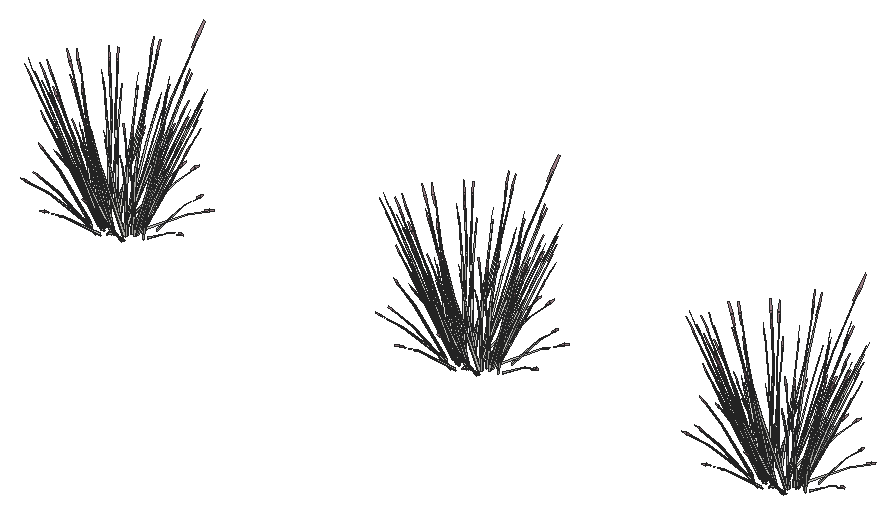
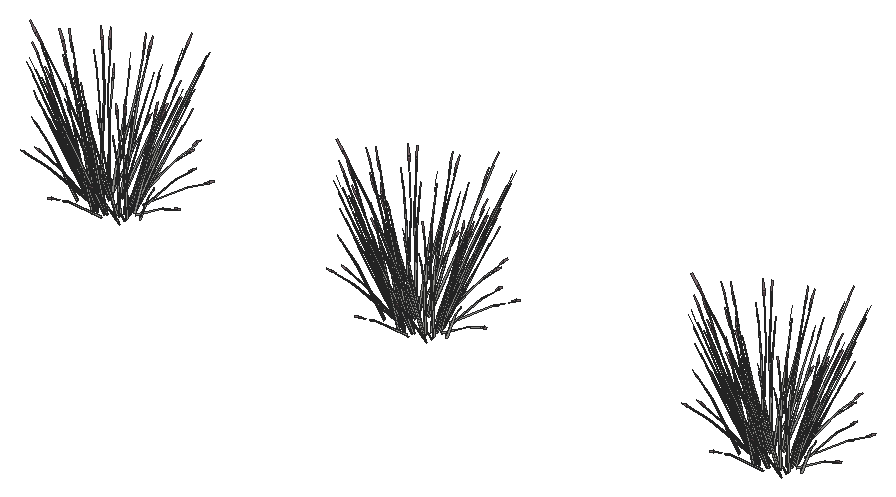
# SketchUp Ruby script. Lengths in millimetres.
U = 1.mm
M = Sketchup.active_model
def pt(a) = Geom::Point3d.new(a.map { |v| v * U })
def face(e, loops, mat)
  f = e.add_face(loops[0].map { |a| pt(a) })
  loops[1..].each { |l| e.add_face(l.map { |a| pt(a) }).erase! }
  f.material = f.back_material = mat if mat
  f
end
# faces: each face lists its corners as indices into pts; further lists are holes
def faces(e, pts, list, mat = nil) = list.each { |f| face(e, (f[0].is_a?(Array) ? f : [f]).map { |l| l.map { |i| pts[i] } }, mat) }
# xy, xz, yz: faces in a plane at the given z, y or x. An outline is a flat list of corners, or four numbers for a rectangle; further outlines are holes
def ring(l) = l.size == 4 ? [[l[0], l[1]], [l[2], l[1]], [l[2], l[3]], [l[0], l[3]]] : l.each_slice(2).to_a
def flat(e, list, mat, &to3) = list.each { |f| face(e, (f[0].is_a?(Array) ? f : [f]).map { |l| ring(l).map { |u, v| to3.(u, v) } }, mat) }
def xy(e, z, list, mat = nil) = flat(e, list, mat) { |x, y| [x, y, z] }
def xz(e, y, list, mat = nil) = flat(e, list, mat) { |x, z| [x, y, z] }
def yz(e, x, list, mat = nil) = flat(e, list, mat) { |y, z| [x, y, z] }
def lines(e, pts, list) = list.each { |a, b| e.add_line(pt(pts[a]), pt(pts[b])) }
# prism: a flat outline (further loops are holes) pulled along v
def prism(e, loops, v, mat = nil)
  f = face(e, loops, mat); d = Geom::Vector3d.new(v.map { |x| x * U })
  f.pushpull(f.normal.samedirection?(d) ? d.length : -d.length)
end
def box(e, o, s, mat = nil) = prism(e, [[o, [o[0] + s[0], o[1], o[2]], [o[0] + s[0], o[1] + s[1], o[2]], [o[0], o[1] + s[1], o[2]]]], [0, 0, s[2]], mat)
def at(x, y, z, deg = 0) = Geom::Transformation.translation(pt([x, y, z])) * Geom::Transformation.rotation(ORIGIN, Z_AXIS, deg.degrees)
def axes(o, x, y, z) = Geom::Transformation.new([*x, 0, *y, 0, *z, 0, *pt(o).to_a, 1])
def part(name) = M.definitions.add(name)
# library, detail: a bought-in or finely detailed component or shape, given as its bounding box
def library(name, o, s) = part(name).tap { |d| box(d.entities, o, s) }
def detail(e, o, s) = box(e.add_group.entities, o, s)
def put(e, d, t, mat = nil) = e.add_instance(d, t).tap { |i| i.material = mat if mat }
def group(e, t, mat = nil) = e.add_group.tap { |g| g.transformation = t; g.material = mat if mat }.entities
root = M.entities
M.materials.add("LightPink_Translucent").color = [144, 107, 117]
M.materials["LightPink_Translucent"].alpha = 0.8
c1 = part("blade")
p = [[54.7,5.3,558.8],[0,4.4,0],[2.3,11.5,0],[55.5,7.8,558.8],[58.2,7.8,558.8],[9.8,11.5,0],
  [62.9,5.7,838.2],[63,6,838.2],[63.4,6,838.2]]
faces(c1.entities,p,[[0,1,2,3],[4,5,2,3],[6,0,3,7],[7,3,4,8]])
c2 = part("seeds")
p = [[7.6,-2.7,35.1],[-0.2,-0.6,40.4],[-0.2,-0.8,0.9],[3.5,-1.8,-1.7],[7.5,-0.8,76.3],[3.7,0.2,78.9]]
faces(c2.entities,p,[[0,1,2,3],[1,0,4,5]],"LightPink_Translucent")
c3 = part("blade with seeds")
put(c3.entities,c1,at(0,0,0))
put(c3.entities,c2,axes([60.9,6.5,787.2],[1.5799,-0.05474,1.17369],[-0.12525,1.92788,0.29478],[-0.07173,-0.02425,1.56792]))
put(root,c3,axes([12521.7,4405.6,127.9],[0.06562,-1.05324,-0.1216],[1.2424,0.02879,-0.67495],[0.4785,0.07316,1.02557]))
put(root,c3,axes([12285.5,4303,127.9],[0.6166,0.93779,-0.1216],[-1.09436,0.46085,-0.67495],[-0.46117,0.12373,1.02557]))
put(root,c3,axes([12518.5,4251,127.9],[-1.34686,-0.05131,-0.1216],[0.03681,-0.97156,-0.67495],[0.09356,-0.37418,1.02557]))
put(root,c3,axes([12556.8,4356.2,127.9],[-0.6166,-0.93779,-0.1216],[1.09436,-0.46085,-0.67495],[0.46117,-0.12373,1.02557]))
put(root,c3,axes([12387.1,4435.7,127.9],[1.19922,-0.48218,-0.1216],[0.58932,0.85579,-0.67495],[0.15822,0.36063,1.02557]))
put(root,c3,axes([12320.7,4253.5,127.9],[-0.06562,1.05324,-0.1216],[-1.2424,-0.02879,-0.67495],[-0.4785,-0.07316,1.02557]))
put(root,c3,axes([12459.5,4434.8,127.9],[0.73026,-0.88648,-0.1216],[1.05755,0.51071,-0.67495],[0.36761,0.25045,1.02557]))
put(root,c3,axes([12286.7,4359.6,127.9],[1.1336,0.57106,-0.1216],[-0.65308,0.827,-0.67495],[-0.32027,0.28747,1.02557]))
put(root,c3,axes([12455.2,4223.5,127.9],[-1.19922,0.48218,-0.1216],[-0.58932,-0.85579,-0.67495],[-0.15822,-0.36063,1.02557]))
put(root,c3,axes([12555.7,4299.5,127.9],[-1.1336,-0.57106,-0.1216],[0.65308,-0.827,-0.67495],[0.32027,-0.28747,1.02557]))
put(root,c3,axes([10242,4389.4,127.9],[0.06562,-1.05324,-0.1216],[1.2424,0.02879,-0.67495],[0.4785,0.07316,1.02557]))
put(root,c3,axes([10005.8,4286.7,127.9],[0.6166,0.93779,-0.1216],[-1.09436,0.46085,-0.67495],[-0.46117,0.12373,1.02557]))
put(root,c3,axes([10238.8,4234.8,127.9],[-1.34686,-0.05131,-0.1216],[0.03681,-0.97156,-0.67495],[0.09356,-0.37418,1.02557]))
put(root,c3,axes([10277.2,4339.9,127.9],[-0.6166,-0.93779,-0.1216],[1.09436,-0.46085,-0.67495],[0.46117,-0.12373,1.02557]))
put(root,c3,axes([10107.5,4419.4,127.9],[1.19922,-0.48218,-0.1216],[0.58932,0.85579,-0.67495],[0.15822,0.36063,1.02557]))
put(root,c3,axes([10041,4237.3,127.9],[-0.06562,1.05324,-0.1216],[-1.2424,-0.02879,-0.67495],[-0.4785,-0.07316,1.02557]))
put(root,c3,axes([10179.9,4418.5,127.9],[0.73026,-0.88648,-0.1216],[1.05755,0.51071,-0.67495],[0.36761,0.25045,1.02557]))
put(root,c3,axes([10007,4343.4,127.9],[1.1336,0.57106,-0.1216],[-0.65308,0.827,-0.67495],[-0.32027,0.28747,1.02557]))
put(root,c3,axes([10175.5,4207.2,127.9],[-1.19922,0.48218,-0.1216],[-0.58932,-0.85579,-0.67495],[-0.15822,-0.36063,1.02557]))
put(root,c3,axes([10276,4283.3,127.9],[-1.1336,-0.57106,-0.1216],[0.65308,-0.827,-0.67495],[0.32027,-0.28747,1.02557]))
put(root,c3,axes([7622,4346,127.9],[0.06562,-1.05324,-0.1216],[1.2424,0.02879,-0.67495],[0.4785,0.07316,1.02557]))
put(root,c3,axes([7385.8,4243.3,127.9],[0.6166,0.93779,-0.1216],[-1.09436,0.46085,-0.67495],[-0.46117,0.12373,1.02557]))
put(root,c3,axes([7618.8,4191.3,127.9],[-1.34686,-0.05131,-0.1216],[0.03681,-0.97156,-0.67495],[0.09356,-0.37418,1.02557]))
put(root,c3,axes([7657.2,4296.5,127.9],[-0.6166,-0.93779,-0.1216],[1.09436,-0.46085,-0.67495],[0.46117,-0.12373,1.02557]))
put(root,c3,axes([7487.5,4376,127.9],[1.19922,-0.48218,-0.1216],[0.58932,0.85579,-0.67495],[0.15822,0.36063,1.02557]))
put(root,c3,axes([7421,4193.8,127.9],[-0.06562,1.05324,-0.1216],[-1.2424,-0.02879,-0.67495],[-0.4785,-0.07316,1.02557]))
put(root,c3,axes([7559.9,4375.1,127.9],[0.73026,-0.88648,-0.1216],[1.05755,0.51071,-0.67495],[0.36761,0.25045,1.02557]))
put(root,c3,axes([7387,4299.9,127.9],[1.1336,0.57106,-0.1216],[-0.65308,0.827,-0.67495],[-0.32027,0.28747,1.02557]))
put(root,c3,axes([7555.5,4163.8,127.9],[-1.19922,0.48218,-0.1216],[-0.58932,-0.85579,-0.67495],[-0.15822,-0.36063,1.02557]))
put(root,c3,axes([7656,4239.9,127.9],[-1.1336,-0.57106,-0.1216],[0.65308,-0.827,-0.67495],[0.32027,-0.28747,1.02557]))
put(root,c3,axes([12480.5,4301.9,113.6],[-1.05895,-0.53811,1.38283],[1.11816,-0.83781,0.59665],[0.34166,0.5049,1.33663]))
put(root,c3,axes([10200.8,4285.7,113.6],[-1.05895,-0.53811,1.38283],[1.11816,-0.83781,0.59665],[0.34166,0.5049,1.33663]))
put(root,c3,axes([7580.9,4242.2,113.6],[-1.05895,-0.53811,1.38283],[1.11816,-0.83781,0.59665],[0.34166,0.5049,1.33663]))
put(root,c3,axes([12252.8,4326.8,119.8],[-0.20012,0.13446,1.74944],[0.01702,0.98243,-0.27667],[-0.45871,0.12776,0.14031]))
put(root,c3,axes([12641.9,4318.8,119.8],[0.17006,-0.15775,1.74944],[-0.21766,-0.96766,-0.27667],[0.42669,-0.18347,0.14031]))
put(root,c3,axes([12549.1,4389.6,119.8],[0.26289,-0.01751,1.74944],[0.72108,-0.8046,-0.27667],[0.46761,0.10621,0.14031]))
put(root,c3,axes([12549.5,4211.8,119.8],[-0.01183,-0.20612,1.74944],[-0.99913,-0.59572,-0.27667],[0.15447,-0.36112,0.14031]))
put(root,c3,axes([12253.6,4419.9,119.8],[-0.03046,0.20495,1.74944],[0.86449,0.71297,-0.27667],[-0.22632,0.33716,0.14031]))
put(root,c3,axes([12380,4484.3,119.8],[0.15534,0.16677,1.74944],[1.25362,0.06552,-0.27667],[0.12606,0.3678,0.14031]))
put(root,c3,axes([12406.8,4166.6,119.8],[-0.18744,-0.14521,1.74944],[-1.25089,0.09206,-0.27667],[-0.19964,-0.34731,0.14031]))
put(root,c3,axes([12302.6,4207.1,119.8],[-0.26368,-0.00731,1.74944],[-0.83946,0.73103,-0.27667],[-0.44791,-0.14937,0.14031]))
put(root,c3,axes([9973.1,4310.5,119.8],[-0.20012,0.13446,1.74944],[0.01702,0.98243,-0.27667],[-0.45871,0.12776,0.14031]))
put(root,c3,axes([10362.2,4302.6,119.8],[0.17006,-0.15775,1.74944],[-0.21766,-0.96766,-0.27667],[0.42669,-0.18347,0.14031]))
put(root,c3,axes([10269.4,4373.4,119.8],[0.26289,-0.01751,1.74944],[0.72108,-0.8046,-0.27667],[0.46761,0.10621,0.14031]))
put(root,c3,axes([10269.9,4195.5,119.8],[-0.01183,-0.20612,1.74944],[-0.99913,-0.59572,-0.27667],[0.15447,-0.36112,0.14031]))
put(root,c3,axes([9974,4403.7,119.8],[-0.03046,0.20495,1.74944],[0.86449,0.71297,-0.27667],[-0.22632,0.33716,0.14031]))
put(root,c3,axes([10100.3,4468.1,119.8],[0.15534,0.16677,1.74944],[1.25362,0.06552,-0.27667],[0.12606,0.3678,0.14031]))
put(root,c3,axes([10127.1,4150.3,119.8],[-0.18744,-0.14521,1.74944],[-1.25089,0.09206,-0.27667],[-0.19964,-0.34731,0.14031]))
put(root,c3,axes([10023,4190.9,119.8],[-0.26368,-0.00731,1.74944],[-0.83946,0.73103,-0.27667],[-0.44791,-0.14937,0.14031]))
put(root,c3,axes([7353.1,4267.1,119.8],[-0.20012,0.13446,1.74944],[0.01702,0.98243,-0.27667],[-0.45871,0.12776,0.14031]))
put(root,c3,axes([7742.2,4259.1,119.8],[0.17006,-0.15775,1.74944],[-0.21766,-0.96766,-0.27667],[0.42669,-0.18347,0.14031]))
put(root,c3,axes([7649.4,4329.9,119.8],[0.26289,-0.01751,1.74944],[0.72108,-0.8046,-0.27667],[0.46761,0.10621,0.14031]))
put(root,c3,axes([7649.9,4152.1,119.8],[-0.01183,-0.20612,1.74944],[-0.99913,-0.59572,-0.27667],[0.15447,-0.36112,0.14031]))
put(root,c3,axes([7354,4360.2,119.8],[-0.03046,0.20495,1.74944],[0.86449,0.71297,-0.27667],[-0.22632,0.33716,0.14031]))
put(root,c3,axes([7480.3,4424.6,119.8],[0.15534,0.16677,1.74944],[1.25362,0.06552,-0.27667],[0.12606,0.3678,0.14031]))
put(root,c3,axes([7507.1,4106.9,119.8],[-0.18744,-0.14521,1.74944],[-1.25089,0.09206,-0.27667],[-0.19964,-0.34731,0.14031]))
put(root,c3,axes([7403,4147.5,119.8],[-0.26368,-0.00731,1.74944],[-0.83946,0.73103,-0.27667],[-0.44791,-0.14937,0.14031]))
put(root,c3,axes([12276.9,4222.9,119.6],[0.09085,0.10335,1.77383],[-0.43798,0.92907,-0.16761],[-0.44357,0.00672,0.31391]))
put(root,c3,axes([12374.2,4154.5,119.6],[-0.02286,0.12414,1.77383],[-1.12758,0.45052,-0.16761],[-0.33182,-0.23029,0.31391]))
put(root,c3,axes([12435.3,4453.4,119.6],[0.00363,-0.12539,1.77383],[1.0502,-0.55319,-0.16761],[0.36479,0.19745,0.31391]))
put(root,c3,axes([12196.3,4352,119.6],[0.1564,0.02778,1.77383],[0.48382,0.91506,-0.16761],[-0.32016,0.24017,0.31391]))
put(root,c3,axes([12626.6,4293.3,119.6],[-0.16006,-0.00787,1.77383],[-0.66468,-0.8428,-0.16761],[0.26693,-0.27711,0.31391]))
put(root,c3,axes([12619.1,4426.9,119.6],[-0.11081,-0.09067,1.77383],[0.2424,-0.97188,-0.16761],[0.43649,-0.06209,0.31391]))
put(root,c3,axes([12251.2,4473.3,119.6],[0.13903,-0.06253,1.77383],[1.14912,0.41591,-0.16761],[-0.027,0.34629,0.31391]))
put(root,c3,axes([12542.8,4193,119.6],[-0.12446,0.07911,1.77383],[-1.21937,-0.26689,-0.16761],[-0.04414,-0.34521,0.31391]))
put(root,c3,axes([9997.2,4206.7,119.6],[0.09085,0.10335,1.77383],[-0.43798,0.92907,-0.16761],[-0.44357,0.00672,0.31391]))
put(root,c3,axes([10094.6,4138.2,119.6],[-0.02286,0.12414,1.77383],[-1.12758,0.45052,-0.16761],[-0.33182,-0.23029,0.31391]))
put(root,c3,axes([10155.6,4437.2,119.6],[0.00363,-0.12539,1.77383],[1.0502,-0.55319,-0.16761],[0.36479,0.19745,0.31391]))
put(root,c3,axes([9916.6,4335.8,119.6],[0.1564,0.02778,1.77383],[0.48382,0.91506,-0.16761],[-0.32016,0.24017,0.31391]))
put(root,c3,axes([10346.9,4277,119.6],[-0.16006,-0.00787,1.77383],[-0.66468,-0.8428,-0.16761],[0.26693,-0.27711,0.31391]))
put(root,c3,axes([10339.5,4410.7,119.6],[-0.11081,-0.09067,1.77383],[0.2424,-0.97188,-0.16761],[0.43649,-0.06209,0.31391]))
put(root,c3,axes([9971.5,4457.1,119.6],[0.13903,-0.06253,1.77383],[1.14912,0.41591,-0.16761],[-0.027,0.34629,0.31391]))
put(root,c3,axes([10263.1,4176.7,119.6],[-0.12446,0.07911,1.77383],[-1.21937,-0.26689,-0.16761],[-0.04414,-0.34521,0.31391]))
put(root,c3,axes([7377.2,4163.2,119.6],[0.09085,0.10335,1.77383],[-0.43798,0.92907,-0.16761],[-0.44357,0.00672,0.31391]))
put(root,c3,axes([7474.6,4094.8,119.6],[-0.02286,0.12414,1.77383],[-1.12758,0.45052,-0.16761],[-0.33182,-0.23029,0.31391]))
put(root,c3,axes([7535.6,4393.8,119.6],[0.00363,-0.12539,1.77383],[1.0502,-0.55319,-0.16761],[0.36479,0.19745,0.31391]))
put(root,c3,axes([7296.6,4292.3,119.6],[0.1564,0.02778,1.77383],[0.48382,0.91506,-0.16761],[-0.32016,0.24017,0.31391]))
put(root,c3,axes([7726.9,4233.6,119.6],[-0.16006,-0.00787,1.77383],[-0.66468,-0.8428,-0.16761],[0.26693,-0.27711,0.31391]))
put(root,c3,axes([7719.5,4367.2,119.6],[-0.11081,-0.09067,1.77383],[0.2424,-0.97188,-0.16761],[0.43649,-0.06209,0.31391]))
put(root,c3,axes([7351.5,4413.6,119.6],[0.13903,-0.06253,1.77383],[1.14912,0.41591,-0.16761],[-0.027,0.34629,0.31391]))
put(root,c3,axes([7643.1,4133.3,119.6],[-0.12446,0.07911,1.77383],[-1.21937,-0.26689,-0.16761],[-0.04414,-0.34521,0.31391]))
put(root,c3,axes([12323.9,4408.2,137.1],[1.34686,0.05131,-0.13498],[-0.03681,0.97156,-0.74919],[-0.09356,0.37418,1.13838]))
put(root,c3,axes([10044.2,4391.9,137.1],[1.34686,0.05131,-0.13498],[-0.03681,0.97156,-0.74919],[-0.09356,0.37418,1.13838]))
put(root,c3,axes([7424.2,4348.5,137.1],[1.34686,0.05131,-0.13498],[-0.03681,0.97156,-0.74919],[-0.09356,0.37418,1.13838]))
put(root,c3,axes([12382.3,4214.4,137.9],[-0.81789,0.99285,-0.13619],[-1.18445,-0.572,-0.75594],[-0.41173,-0.28051,1.14864]))
put(root,c3,axes([10102.6,4198.2,137.9],[-0.81789,0.99285,-0.13619],[-1.18445,-0.572,-0.75594],[-0.41173,-0.28051,1.14864]))
put(root,c3,axes([7482.6,4154.7,137.9],[-0.81789,0.99285,-0.13619],[-1.18445,-0.572,-0.75594],[-0.41173,-0.28051,1.14864]))
put(root,c3,axes([12375.9,4216.1,120.2],[0.55698,-0.6579,0.0643],[0.79316,0.38303,0.50621],[-0.25643,-0.21093,0.77189]))
put(root,c3,axes([12387.8,4445.5,120.2],[-0.90301,0.35198,0.0643],[-0.44199,-0.64184,0.50621],[0.08721,0.28293,0.77189]))
put(root,c3,axes([12566.2,4294.2,120.2],[0.8413,0.43556,0.0643],[-0.48981,0.62025,0.50621],[0.26973,-0.20053,0.77189]))
put(root,c3,axes([12569.4,4355.6,120.2],[0.4501,0.70615,0.0643],[-0.82077,0.34564,0.50621],[0.36181,-0.0682,0.77189]))
put(root,c3,axes([12309.5,4249,120.2],[0.06171,-0.78753,0.0643],[0.9318,0.02159,0.50621],[-0.35694,-0.08241,0.77189]))
put(root,c3,axes([12524.1,4242.2,120.2],[1.00708,0.04826,0.0643],[-0.02761,0.72867,0.50621],[0.10538,-0.27912,0.77189]))
put(root,c3,axes([12532.9,4410.1,120.2],[-0.06171,0.78753,0.0643],[-0.9318,-0.02159,0.50621],[0.35694,0.08241,0.77189]))
put(root,c3,axes([12276.1,4364.9,120.2],[-0.8413,-0.43556,0.0643],[0.48981,-0.62025,0.50621],[-0.26973,0.20053,0.77189]))
put(root,c3,axes([12454.5,4213.7,120.2],[0.90301,-0.35198,0.0643],[0.44199,0.64184,0.50621],[-0.08721,-0.28293,0.77189]))
put(root,c3,axes([12272.9,4303.5,120.2],[-0.4501,-0.70615,0.0643],[0.82077,-0.34564,0.50621],[-0.36181,0.0682,0.77189]))
put(root,c3,axes([12466.4,4443,120.2],[-0.55698,0.6579,0.0643],[-0.79316,-0.38303,0.50621],[0.25643,0.21093,0.77189]))
put(root,c3,axes([12318.2,4416.9,120.2],[-1.00708,-0.04826,0.0643],[0.02761,-0.72867,0.50621],[-0.10538,0.27912,0.77189]))
put(root,c3,axes([10096.2,4199.9,120.2],[0.55698,-0.6579,0.0643],[0.79316,0.38303,0.50621],[-0.25643,-0.21093,0.77189]))
put(root,c3,axes([10108.1,4429.3,120.2],[-0.90301,0.35198,0.0643],[-0.44199,-0.64184,0.50621],[0.08721,0.28293,0.77189]))
put(root,c3,axes([10286.5,4278,120.2],[0.8413,0.43556,0.0643],[-0.48981,0.62025,0.50621],[0.26973,-0.20053,0.77189]))
put(root,c3,axes([10289.7,4339.4,120.2],[0.4501,0.70615,0.0643],[-0.82077,0.34564,0.50621],[0.36181,-0.0682,0.77189]))
put(root,c3,axes([10029.8,4232.8,120.2],[0.06171,-0.78753,0.0643],[0.9318,0.02159,0.50621],[-0.35694,-0.08241,0.77189]))
put(root,c3,axes([10244.5,4226,120.2],[1.00708,0.04826,0.0643],[-0.02761,0.72867,0.50621],[0.10538,-0.27912,0.77189]))
put(root,c3,axes([10253.2,4393.9,120.2],[-0.06171,0.78753,0.0643],[-0.9318,-0.02159,0.50621],[0.35694,0.08241,0.77189]))
put(root,c3,axes([9996.4,4348.7,120.2],[-0.8413,-0.43556,0.0643],[0.48981,-0.62025,0.50621],[-0.26973,0.20053,0.77189]))
put(root,c3,axes([10174.8,4197.4,120.2],[0.90301,-0.35198,0.0643],[0.44199,0.64184,0.50621],[-0.08721,-0.28293,0.77189]))
put(root,c3,axes([9993.3,4287.3,120.2],[-0.4501,-0.70615,0.0643],[0.82077,-0.34564,0.50621],[-0.36181,0.0682,0.77189]))
put(root,c3,axes([10186.7,4426.8,120.2],[-0.55698,0.6579,0.0643],[-0.79316,-0.38303,0.50621],[0.25643,0.21093,0.77189]))
put(root,c3,axes([10038.5,4400.7,120.2],[-1.00708,-0.04826,0.0643],[0.02761,-0.72867,0.50621],[-0.10538,0.27912,0.77189]))
put(root,c3,axes([7476.2,4156.5,120.2],[0.55698,-0.6579,0.0643],[0.79316,0.38303,0.50621],[-0.25643,-0.21093,0.77189]))
put(root,c3,axes([7488.2,4385.8,120.2],[-0.90301,0.35198,0.0643],[-0.44199,-0.64184,0.50621],[0.08721,0.28293,0.77189]))
put(root,c3,axes([7666.5,4234.5,120.2],[0.8413,0.43556,0.0643],[-0.48981,0.62025,0.50621],[0.26973,-0.20053,0.77189]))
put(root,c3,axes([7669.7,4296,120.2],[0.4501,0.70615,0.0643],[-0.82077,0.34564,0.50621],[0.36181,-0.0682,0.77189]))
put(root,c3,axes([7409.8,4189.4,120.2],[0.06171,-0.78753,0.0643],[0.9318,0.02159,0.50621],[-0.35694,-0.08241,0.77189]))
put(root,c3,axes([7624.5,4182.5,120.2],[1.00708,0.04826,0.0643],[-0.02761,0.72867,0.50621],[0.10538,-0.27912,0.77189]))
put(root,c3,axes([7633.2,4350.4,120.2],[-0.06171,0.78753,0.0643],[-0.9318,-0.02159,0.50621],[0.35694,0.08241,0.77189]))
put(root,c3,axes([7376.4,4305.3,120.2],[-0.8413,-0.43556,0.0643],[0.48981,-0.62025,0.50621],[-0.26973,0.20053,0.77189]))
put(root,c3,axes([7554.8,4154,120.2],[0.90301,-0.35198,0.0643],[0.44199,0.64184,0.50621],[-0.08721,-0.28293,0.77189]))
put(root,c3,axes([7373.3,4243.8,120.2],[-0.4501,-0.70615,0.0643],[0.82077,-0.34564,0.50621],[-0.36181,0.0682,0.77189]))
put(root,c3,axes([7566.7,4383.3,120.2],[-0.55698,0.6579,0.0643],[-0.79316,-0.38303,0.50621],[0.25643,0.21093,0.77189]))
put(root,c3,axes([7418.5,4357.2,120.2],[-1.00708,-0.04826,0.0643],[0.02761,-0.72867,0.50621],[-0.10538,0.27912,0.77189]))
put(root,c3,axes([12446.4,4215.4,120.2],[1.20755,0.27075,0.48003],[-0.41292,0.89013,0.3958],[-0.07257,-0.35005,0.9933]))
put(root,c3,axes([12535,4403.7,120.2],[-0.90362,0.68241,0.48003],[-0.77932,-0.72471,0.3958],[0.42395,0.12588,0.9933]))
put(root,c3,axes([12567.2,4349.3,120.2],[-0.34623,0.9443,0.48003],[-1.13828,-0.3229,0.3958],[0.44763,-0.05675,0.9933]))
put(root,c3,axes([12282.1,4369.6,120.2],[-0.30393,-0.95317,0.48003],[1.19224,-0.16542,0.3958],[-0.35138,0.22417,0.9933]))
put(root,c3,axes([12326.3,4418.6,120.2],[-0.87265,-0.70663,0.48003],[0.92674,-0.60943,0.3958],[-0.16097,0.33153,0.9933]))
put(root,c3,axes([12516,4240.5,120.2],[0.87265,0.70663,0.48003],[-0.92674,0.60943,0.3958],[0.16097,-0.33153,0.9933]))
put(root,c3,axes([12275.1,4309.9,120.2],[0.34623,-0.9443,0.48003],[1.13828,0.3229,0.3958],[-0.44763,0.05675,0.9933]))
put(root,c3,axes([12560.2,4289.5,120.2],[0.30393,0.95317,0.48003],[-1.19224,0.16542,0.3958],[0.35138,-0.22417,0.9933]))
put(root,c3,axes([12472.4,4438.3,120.2],[-1.21888,0.23767,0.48003],[-0.21154,-0.93233,0.3958],[0.28666,0.27478,0.9933]))
put(root,c3,axes([10166.7,4199.1,120.2],[1.20755,0.27075,0.48003],[-0.41292,0.89013,0.3958],[-0.07257,-0.35005,0.9933]))
put(root,c3,axes([10255.3,4387.5,120.2],[-0.90362,0.68241,0.48003],[-0.77932,-0.72471,0.3958],[0.42395,0.12588,0.9933]))
put(root,c3,axes([10287.5,4333,120.2],[-0.34623,0.9443,0.48003],[-1.13828,-0.3229,0.3958],[0.44763,-0.05675,0.9933]))
put(root,c3,axes([10002.4,4353.4,120.2],[-0.30393,-0.95317,0.48003],[1.19224,-0.16542,0.3958],[-0.35138,0.22417,0.9933]))
put(root,c3,axes([10046.6,4402.4,120.2],[-0.87265,-0.70663,0.48003],[0.92674,-0.60943,0.3958],[-0.16097,0.33153,0.9933]))
put(root,c3,axes([10236.3,4224.3,120.2],[0.87265,0.70663,0.48003],[-0.92674,0.60943,0.3958],[0.16097,-0.33153,0.9933]))
put(root,c3,axes([9995.5,4293.6,120.2],[0.34623,-0.9443,0.48003],[1.13828,0.3229,0.3958],[-0.44763,0.05675,0.9933]))
put(root,c3,axes([10280.5,4273.3,120.2],[0.30393,0.95317,0.48003],[-1.19224,0.16542,0.3958],[0.35138,-0.22417,0.9933]))
put(root,c3,axes([10192.7,4422.1,120.2],[-1.21888,0.23767,0.48003],[-0.21154,-0.93233,0.3958],[0.28666,0.27478,0.9933]))
put(root,c3,axes([7546.7,4155.7,120.2],[1.20755,0.27075,0.48003],[-0.41292,0.89013,0.3958],[-0.07257,-0.35005,0.9933]))
put(root,c3,axes([7635.4,4344,120.2],[-0.90362,0.68241,0.48003],[-0.77932,-0.72471,0.3958],[0.42395,0.12588,0.9933]))
put(root,c3,axes([7667.5,4289.6,120.2],[-0.34623,0.9443,0.48003],[-1.13828,-0.3229,0.3958],[0.44763,-0.05675,0.9933]))
put(root,c3,axes([7382.4,4309.9,120.2],[-0.30393,-0.95317,0.48003],[1.19224,-0.16542,0.3958],[-0.35138,0.22417,0.9933]))
put(root,c3,axes([7426.7,4358.9,120.2],[-0.87265,-0.70663,0.48003],[0.92674,-0.60943,0.3958],[-0.16097,0.33153,0.9933]))
put(root,c3,axes([7616.3,4180.8,120.2],[0.87265,0.70663,0.48003],[-0.92674,0.60943,0.3958],[0.16097,-0.33153,0.9933]))
put(root,c3,axes([7375.5,4250.2,120.2],[0.34623,-0.9443,0.48003],[1.13828,0.3229,0.3958],[-0.44763,0.05675,0.9933]))
put(root,c3,axes([7660.5,4229.8,120.2],[0.30393,0.95317,0.48003],[-1.19224,0.16542,0.3958],[0.35138,-0.22417,0.9933]))
put(root,c3,axes([7572.7,4378.6,120.2],[-1.21888,0.23767,0.48003],[-0.21154,-0.93233,0.3958],[0.28666,0.27478,0.9933]))
put(root,c3,axes([12396.3,4427.1,128.3],[0.36946,-0.79643,0.35414],[1.07787,0.23229,-0.4572],[0.09883,0.32066,0.87481]))
put(root,c3,axes([12446,4232,128.3],[-0.36946,0.79643,0.35414],[-1.07787,-0.23229,-0.4572],[-0.09883,-0.32066,0.87481]))
put(root,c3,axes([12516.8,4395.2,128.3],[-0.69728,-0.64842,0.35414],[0.79619,-0.61382,-0.4572],[0.40453,0.09339,0.87481]))
put(root,c3,axes([12545.9,4349,128.3],[-1.01846,-0.28891,0.35414],[0.29705,-0.84289,-0.4572],[0.41005,-0.07729,0.87481]))
put(root,c3,axes([12325.5,4264,128.3],[0.69728,0.64842,0.35414],[-0.79619,0.61382,-0.4572],[-0.40453,-0.09339,0.87481]))
put(root,c3,axes([12337.3,4404.4,128.3],[0.82919,-0.54528,0.35414],[0.78493,0.62262,-0.4572],[-0.11943,0.31634,0.87481]))
put(root,c3,axes([12300.7,4361.5,128.3],[1.06674,-0.14801,0.35414],[0.28168,0.84611,-0.4572],[-0.30569,0.22726,0.87481]))
put(root,c3,axes([12462.1,4423.8,128.3],[-0.18927,-0.83419,0.35414],[1.08199,-0.22027,-0.4572],[0.29062,0.23905,0.87481]))
put(root,c3,axes([12541.6,4297.6,128.3],[-1.06674,0.14801,0.35414],[-0.28168,-0.84611,-0.4572],[0.30569,-0.22726,0.87481]))
put(root,c3,axes([12296.4,4310.2,128.3],[1.01846,0.28891,0.35414],[-0.29705,0.84289,-0.4572],[-0.41005,0.07729,0.87481]))
put(root,c3,axes([12505,4254.8,128.3],[-0.82919,0.54528,0.35414],[-0.78493,-0.62262,-0.4572],[0.11943,-0.31634,0.87481]))
put(root,c3,axes([12380.3,4235.4,128.3],[0.18927,0.83419,0.35414],[-1.08199,0.22027,-0.4572],[-0.29062,-0.23905,0.87481]))
put(root,c3,axes([10116.7,4410.9,128.3],[0.36946,-0.79643,0.35414],[1.07787,0.23229,-0.4572],[0.09883,0.32066,0.87481]))
put(root,c3,axes([10166.3,4215.8,128.3],[-0.36946,0.79643,0.35414],[-1.07787,-0.23229,-0.4572],[-0.09883,-0.32066,0.87481]))
put(root,c3,axes([10237.1,4378.9,128.3],[-0.69728,-0.64842,0.35414],[0.79619,-0.61382,-0.4572],[0.40453,0.09339,0.87481]))
put(root,c3,axes([10266.3,4332.8,128.3],[-1.01846,-0.28891,0.35414],[0.29705,-0.84289,-0.4572],[0.41005,-0.07729,0.87481]))
put(root,c3,axes([10045.8,4247.7,128.3],[0.69728,0.64842,0.35414],[-0.79619,0.61382,-0.4572],[-0.40453,-0.09339,0.87481]))
put(root,c3,axes([10057.6,4388.1,128.3],[0.82919,-0.54528,0.35414],[0.78493,0.62262,-0.4572],[-0.11943,0.31634,0.87481]))
put(root,c3,axes([10021,4345.3,128.3],[1.06674,-0.14801,0.35414],[0.28168,0.84611,-0.4572],[-0.30569,0.22726,0.87481]))
put(root,c3,axes([10182.4,4407.5,128.3],[-0.18927,-0.83419,0.35414],[1.08199,-0.22027,-0.4572],[0.29062,0.23905,0.87481]))
put(root,c3,axes([10262,4281.4,128.3],[-1.06674,0.14801,0.35414],[-0.28168,-0.84611,-0.4572],[0.30569,-0.22726,0.87481]))
put(root,c3,axes([10016.7,4293.9,128.3],[1.01846,0.28891,0.35414],[-0.29705,0.84289,-0.4572],[-0.41005,0.07729,0.87481]))
put(root,c3,axes([10225.4,4238.5,128.3],[-0.82919,0.54528,0.35414],[-0.78493,-0.62262,-0.4572],[0.11943,-0.31634,0.87481]))
put(root,c3,axes([10100.6,4219.1,128.3],[0.18927,0.83419,0.35414],[-1.08199,0.22027,-0.4572],[-0.29062,-0.23905,0.87481]))
put(root,c3,axes([7496.7,4367.5,128.3],[0.36946,-0.79643,0.35414],[1.07787,0.23229,-0.4572],[0.09883,0.32066,0.87481]))
put(root,c3,axes([7546.3,4172.3,128.3],[-0.36946,0.79643,0.35414],[-1.07787,-0.23229,-0.4572],[-0.09883,-0.32066,0.87481]))
put(root,c3,axes([7617.1,4335.5,128.3],[-0.69728,-0.64842,0.35414],[0.79619,-0.61382,-0.4572],[0.40453,0.09339,0.87481]))
put(root,c3,axes([7646.3,4289.3,128.3],[-1.01846,-0.28891,0.35414],[0.29705,-0.84289,-0.4572],[0.41005,-0.07729,0.87481]))
put(root,c3,axes([7425.8,4204.3,128.3],[0.69728,0.64842,0.35414],[-0.79619,0.61382,-0.4572],[-0.40453,-0.09339,0.87481]))
put(root,c3,axes([7437.6,4344.7,128.3],[0.82919,-0.54528,0.35414],[0.78493,0.62262,-0.4572],[-0.11943,0.31634,0.87481]))
put(root,c3,axes([7401,4301.9,128.3],[1.06674,-0.14801,0.35414],[0.28168,0.84611,-0.4572],[-0.30569,0.22726,0.87481]))
put(root,c3,axes([7562.4,4364.1,128.3],[-0.18927,-0.83419,0.35414],[1.08199,-0.22027,-0.4572],[0.29062,0.23905,0.87481]))
put(root,c3,axes([7642,4237.9,128.3],[-1.06674,0.14801,0.35414],[-0.28168,-0.84611,-0.4572],[0.30569,-0.22726,0.87481]))
put(root,c3,axes([7396.7,4250.5,128.3],[1.01846,0.28891,0.35414],[-0.29705,0.84289,-0.4572],[-0.41005,0.07729,0.87481]))
put(root,c3,axes([7605.4,4195.1,128.3],[-0.82919,0.54528,0.35414],[-0.78493,-0.62262,-0.4572],[0.11943,-0.31634,0.87481]))
put(root,c3,axes([7480.6,4175.7,128.3],[0.18927,0.83419,0.35414],[-1.08199,0.22027,-0.4572],[-0.29062,-0.23905,0.87481]))
put(root,c3,axes([12396,4443.8,128.6],[-1.20755,-0.27075,0.53283],[0.41292,-0.89013,0.43934],[0.07257,0.35005,1.10256]))
put(root,c3,axes([10116.3,4427.5,128.6],[-1.20755,-0.27075,0.53283],[0.41292,-0.89013,0.43934],[0.07257,0.35005,1.10256]))
put(root,c3,axes([7496.3,4384.1,128.6],[-1.20755,-0.27075,0.53283],[0.41292,-0.89013,0.43934],[0.07257,0.35005,1.10256]))
put(root,c3,axes([12297.7,4249.2,129.4],[1.01205,-0.7643,0.53763],[0.87284,0.81167,0.4433],[-0.47482,-0.14098,1.11249]))
put(root,c3,axes([12367.9,4210.4,129.4],[1.36515,-0.26619,0.53763],[0.23692,1.04421,0.4433],[-0.32106,-0.30775,1.11249]))
put(root,c3,axes([10018.1,4232.9,129.4],[1.01205,-0.7643,0.53763],[0.87284,0.81167,0.4433],[-0.47482,-0.14098,1.11249]))
put(root,c3,axes([10088.2,4194.2,129.4],[1.36515,-0.26619,0.53763],[0.23692,1.04421,0.4433],[-0.32106,-0.30775,1.11249]))
put(root,c3,axes([7398.1,4189.5,129.4],[1.01205,-0.7643,0.53763],[0.87284,0.81167,0.4433],[-0.47482,-0.14098,1.11249]))
put(root,c3,axes([7468.3,4150.7,129.4],[1.36515,-0.26619,0.53763],[0.23692,1.04421,0.4433],[-0.32106,-0.30775,1.11249]))
put(root,c3,axes([12433.2,4499.3,143.4],[0.84686,-0.59414,-0.06488],[0.77596,0.65071,-0.29416],[0.05463,0.18438,0.97024]))
put(root,c3,axes([12239.2,4422.6,143.4],[1.08141,0.27645,-0.06488],[-0.33265,0.85086,-0.29416],[-0.17688,0.12919,0.97024]))
put(root,c3,axes([10153.5,4483.1,143.4],[0.84686,-0.59414,-0.06488],[0.77596,0.65071,-0.29416],[0.05463,0.18438,0.97024]))
put(root,c3,axes([9959.5,4406.3,143.4],[1.08141,0.27645,-0.06488],[-0.33265,0.85086,-0.29416],[-0.17688,0.12919,0.97024]))
put(root,c3,axes([7533.5,4439.6,143.4],[0.84686,-0.59414,-0.06488],[0.77596,0.65071,-0.29416],[0.05463,0.18438,0.97024]))
put(root,c3,axes([7339.5,4362.9,143.4],[1.08141,0.27645,-0.06488],[-0.33265,0.85086,-0.29416],[-0.17688,0.12919,0.97024]))
